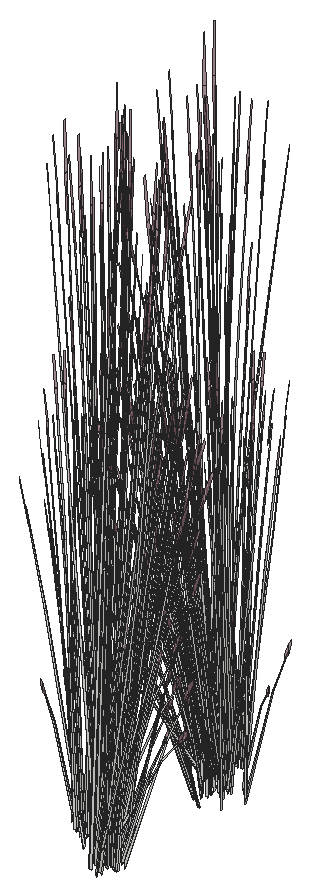
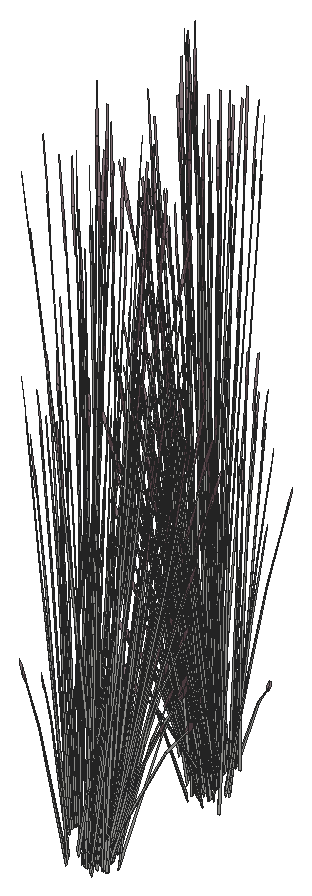
# SketchUp Ruby script. Lengths in inches.
U = 1.inch
M = Sketchup.active_model
def pt(a) = Geom::Point3d.new(a.map { |v| v * U })
def face(e, loops, mat)
  f = e.add_face(loops[0].map { |a| pt(a) })
  loops[1..].each { |l| e.add_face(l.map { |a| pt(a) }).erase! }
  f.material = f.back_material = mat if mat
  f
end
# faces: each face lists its corners as indices into pts; further lists are holes
def faces(e, pts, list, mat = nil) = list.each { |f| face(e, (f[0].is_a?(Array) ? f : [f]).map { |l| l.map { |i| pts[i] } }, mat) }
# xy, xz, yz: faces in a plane at the given z, y or x. An outline is a flat list of corners, or four numbers for a rectangle; further outlines are holes
def ring(l) = l.size == 4 ? [[l[0], l[1]], [l[2], l[1]], [l[2], l[3]], [l[0], l[3]]] : l.each_slice(2).to_a
def flat(e, list, mat, &to3) = list.each { |f| face(e, (f[0].is_a?(Array) ? f : [f]).map { |l| ring(l).map { |u, v| to3.(u, v) } }, mat) }
def xy(e, z, list, mat = nil) = flat(e, list, mat) { |x, y| [x, y, z] }
def xz(e, y, list, mat = nil) = flat(e, list, mat) { |x, z| [x, y, z] }
def yz(e, x, list, mat = nil) = flat(e, list, mat) { |y, z| [x, y, z] }
def lines(e, pts, list) = list.each { |a, b| e.add_line(pt(pts[a]), pt(pts[b])) }
# prism: a flat outline (further loops are holes) pulled along v
def prism(e, loops, v, mat = nil)
  f = face(e, loops, mat); d = Geom::Vector3d.new(v.map { |x| x * U })
  f.pushpull(f.normal.samedirection?(d) ? d.length : -d.length)
end
def box(e, o, s, mat = nil) = prism(e, [[o, [o[0] + s[0], o[1], o[2]], [o[0] + s[0], o[1] + s[1], o[2]], [o[0], o[1] + s[1], o[2]]]], [0, 0, s[2]], mat)
def at(x, y, z, deg = 0) = Geom::Transformation.translation(pt([x, y, z])) * Geom::Transformation.rotation(ORIGIN, Z_AXIS, deg.degrees)
def axes(o, x, y, z) = Geom::Transformation.new([*x, 0, *y, 0, *z, 0, *pt(o).to_a, 1])
def part(name) = M.definitions.add(name)
# library, detail: a bought-in or finely detailed component or shape, given as its bounding box
def library(name, o, s) = part(name).tap { |d| box(d.entities, o, s) }
def detail(e, o, s) = box(e.add_group.entities, o, s)
def put(e, d, t, mat = nil) = e.add_instance(d, t).tap { |i| i.material = mat if mat }
def group(e, t, mat = nil) = e.add_group.tap { |g| g.transformation = t; g.material = mat if mat }.entities
root = M.entities
M.materials.add("LightPink_Translucent").color = [144, 107, 117]
M.materials["LightPink_Translucent"].alpha = 0.75
c1 = part("blade")
p = [[2.15,0.21,22],[0,0.17,0],[0.09,0.45,0],[2.18,0.31,22],[2.29,0.31,22],[0.38,0.45,0],
  [2.48,0.24,33],[2.49,0.24,33],[2.48,0.22,33]]
faces(c1.entities,p,[[0,1,2,3],[4,5,2,3],[6,3,4,7],[8,0,3,6]])
c2 = part("seeds")
p = [[0.3,-0.1,1.38],[-0.01,-0.03,1.59],[-0.01,-0.03,0.03],[0.14,-0.07,-0.07],[0.29,-0.03,3],[0.15,0.01,3.11]]
faces(c2.entities,p,[[0,1,2,3],[1,0,4,5]],"LightPink_Translucent")
c3 = part("blade with seeds")
put(c3.entities,c1,at(0,0,0))
put(c3.entities,c2,axes([2.4,0.25,30.99],[1.5799,-0.05474,1.17369],[-0.12525,1.92788,0.29478],[-0.07173,-0.02425,1.56792]))
put(root,c3,axes([330.96,440.47,1400.67],[-0.35635,0.30962,-0.29095],[-0.23697,-0.43749,-0.50002],[-0.08792,-0.04443,1.59708]))
put(root,c3,axes([331.74,438.73,1400.47],[-0.37926,0.12378,0.17642],[-0.09365,-0.46065,0.35086],[0.03382,0.06712,1.60407]))
put(root,c3,axes([331.98,439.7,1401.875],[-0.14639,0.01056,1.71376],[0.09712,-0.45778,0.13857],[0.20862,0.02831,0.73262]))
put(root,c3,axes([332.17,438.71,1400.03],[0.08291,0.40636,-0.30978],[-0.32928,0.11539,0.30978],[0.06638,0.04686,1.38974]))
put(root,c3,axes([332.73,440.33,1402.73],[0.12963,0.31798,0.0643],[-0.23638,0.15564,0.50621],[0.1042,-0.03071,0.77189]))
put(root,c3,axes([331.5,439.62,1400.38],[-0.44609,-0.09826,0.49198],[0.09078,-0.55493,0.19306],[0.06519,0.05359,1.70813]))
put(root,c3,axes([332.71,440.22,1402.73],[-0.09971,0.42522,0.48003],[-0.32782,-0.1454,0.3958],[0.12892,-0.02555,0.9933]))
put(root,c3,axes([331.15,440.99,1400.2],[-0.11516,-0.40207,0],[0.32884,-0.1408,0],[0,0,1.54371]))
put(root,c3,axes([330.93,440.61,1400.62],[-0.06809,0.4162,0.1448],[-0.33266,-0.07225,-0.41347],[-0.06054,-0.04274,1.26744]))
put(root,c3,axes([329.64,439.53,1403.05],[0.29332,0.1301,0.35414],[-0.08555,0.37955,-0.4572],[-0.11809,0.0348,0.87481]))
put(root,c3,axes([331.58,440.93,1400.18],[0.37054,-0.15823,-0.19198],[0.1302,0.45581,0.00008],[0.0409,-0.01749,1.73897]))
put(root,c3,axes([331.71,441.12,1400.47],[0.10196,-0.46348,0.17642],[0.3731,0.13116,0.35086],[-0.06445,0.00226,1.60407]))
put(root,c3,axes([331.62,440.07,1400.21],[0.24637,0.30123,0],[-0.24637,0.30123,0],[0,0,1.69266]))
put(root,c3,axes([330.22,439.51,1401.34],[0.10032,-0.06746,1.77064],[0.0346,0.47103,0.13857],[-0.2173,0.0625,0.63284]))
put(root,c3,axes([332.29,439.94,1400.47],[-0.2773,-0.3397,0.17642],[0.27945,-0.32949,0.35086],[-0.03063,0.06937,1.60407]))
put(root,c3,axes([331.78,439.43,1400.06],[0.36714,0.07646,-0.62353],[-0.07747,0.47163,-0.16365],[0.10956,0.05715,1.37633]))
put(root,c3,axes([333.4,440.25,1400.77],[-0.21807,0.07699,1.1486],[0.10265,-0.31819,0.84392],[0.11568,0.02177,0.25299]))
put(root,c3,axes([331.07,441.17,1400.2],[-0.35581,-0.20937,0],[0.17124,-0.43505,0],[0,0,1.62707]))
put(root,c3,axes([331.36,440.61,1400.46],[-0.34464,-0.37536,-0.25192],[0.29,-0.42149,0.5513],[-0.0928,0.04391,1.68216]))
put(root,c3,axes([330.45,441.33,1400.48],[0.33032,0.23318,0.49651],[-0.19744,0.41812,0],[-0.07523,-0.05311,1.57504]))
put(root,c3,axes([331.62,439.72,1400.72],[0.17124,-0.42022,0.44739],[0.35581,0.20224,-0.21531],[0,0.09687,1.43643]))
put(root,c3,axes([333.3,441.6,1402.71],[-0.03191,-0.04083,1.77383],[0.06981,-0.43764,-0.16761],[0.12571,-0.02796,0.31391]))
put(root,c3,axes([329.14,439.82,1402.72],[-0.05763,0.06055,1.74944],[0.0049,0.44239,-0.27667],[-0.13211,0.05753,0.14031]))
put(root,c3,axes([331.55,439.96,1400.29],[0,0.53934,-0.05637],[-0.44133,0,0],[0,0.01695,1.79368]))
put(root,c3,axes([329.53,439.76,1402.68],[-0.09562,0.42421,-0.51099],[-0.32782,-0.1454,-0.3958],[-0.13199,0.0389,0.97773]))
put(root,c3,axes([329.51,439.4,1403.03],[0.17758,0.42229,-0.1216],[-0.31518,0.20752,-0.67495],[-0.13282,0.05572,1.02557]))
put(root,c3,axes([331.58,439.58,1400.21],[0.21202,0.39143,-0.44739],[-0.32115,0.27564,0.21531],[0.06861,0.04843,1.43643]))
put(root,c3,axes([333.02,441.23,1401.93],[-0.06755,-0.39203,-0.03492],[0.31928,-0.09013,-0.15832],[0.06667,0.02485,0.52218]))
put(root,c3,axes([330.26,441.58,1400.375],[-0.22066,0.46731,0],[-0.36918,-0.26061,-0.51607],[-0.08408,-0.05936,1.63711]))
put(root,c3,axes([332.19,441.22,1403.03],[0.0189,-0.47427,-0.1216],[0.35781,0.01296,-0.67495],[0.13781,0.03295,1.02557]))
put(root,c3,axes([332.52,439.95,1400.48],[0,-0.46636,0.49651],[0.39487,0,0],[0,0.10622,1.57504]))
put(root,c3,axes([331.53,440.3,1400.72],[0.38326,-0.02879,0.44739],[0.03466,0.47788,-0.21531],[-0.06861,0.04843,1.43643]))
put(root,c3,axes([331.77,439.82,1400.62],[0.32884,-0.136,0.1448],[0.11516,0.38837,-0.41347],[0,0.08547,1.26744]))
put(root,c3,axes([332.14,441.03,1403.05],[-0.20082,-0.29199,0.35414],[0.2293,-0.2764,-0.4572],[0.1165,0.04206,0.87481]))
put(root,c3,axes([331.1875,440.53,1400.21],[-0.38326,0.02879,-0.44739],[-0.03466,-0.47788,0.21531],[-0.06861,0.04843,1.43643]))
put(root,c3,axes([332.99,440.76,1400.59],[-0.085,-0.1147,1.43002],[0.1106,-0.37943,-0.30754],[0.17198,0.0514,0.61141]))
put(root,c3,axes([331.47,441.18,1400.2],[0.35581,0.20937,0],[-0.17124,0.43505,0],[0,0,1.74954]))
put(root,c3,axes([332.5,440.9375,1402.72],[0.07571,-0.00789,1.74944],[0.20767,-0.36231,-0.27667],[0.13467,0.04783,0.14031]))
put(root,c3,axes([331.61,441.64,1400.19],[-0.21791,-0.46895,-0.05142],[0.36918,-0.26061,0.51607],[-0.09097,0.04465,1.6363]))
put(root,c3,axes([331.53,440.51,1400.62],[0.26075,0.2802,0.1448],[-0.2175,0.31612,-0.41347],[-0.06054,0.04274,1.26744]))
put(root,c3,axes([329.47,440.58,1402.73],[-0.08753,-0.42921,0.48003],[0.34336,-0.07449,0.3958],[-0.1012,0.10094,0.9933]))
put(root,c3,axes([329.41,440.5,1402.73],[-0.2423,-0.19613,0.0643],[0.14107,-0.2793,0.50621],[-0.07768,0.0903,0.77189]))
put(root,c3,axes([329.52,439.98,1401.875],[0.12246,-0.09864,1.71376],[0.1031,0.45582,0.13857],[-0.19225,0.10302,0.73262]))
put(root,c3,axes([332.21,440.99,1402.98],[0.35281,0.01123,-0.71045],[-0.0237,0.47284,0.08574],[0.14947,0.0499,1.00501]))
put(root,c3,axes([331.8125,441.37,1400.48],[0.33032,-0.23318,0.49651],[0.19744,0.41812,0],[-0.07523,0.05311,1.57504]))
put(root,c3,axes([331.34,441,1400.29],[0.15345,0.53576,-0.06012],[-0.43845,0.18773,0],[0.00536,0.01871,1.72173]))
put(root,c3,axes([331.51,441.58,1400.03],[-0.32928,-0.11539,-0.30978],[0.08291,-0.40636,0.30978],[-0.06638,0.04686,1.38974]))
put(root,c3,axes([329.14,440.76,1400.59],[0.12266,0.03828,1.43002],[0.07906,0.39104,-0.30754],[-0.16661,0.0732,0.61141]))
put(root,c3,axes([329.6875,440.4375,1403.05],[0.30722,-0.06665,0.35414],[0.08112,0.381,-0.4572],[-0.08804,0.10234,0.87481]))
put(root,c3,axes([332.78,440.03,1400.375],[0.44133,0,0],[0,0.52122,-0.51607],[0,0.11871,1.63711]))
put(root,c3,axes([328.5,440.27,1402.71],[0.04504,0.01251,1.77383],[0.13934,0.41205,-0.16761],[-0.0922,0.10815,0.31391]))
put(root,c3,axes([332.61,440.3,1400.2],[-0.44111,-0.00373,-0.04976],[0,-0.52122,0.49943],[-0.01386,0.11865,1.58352]))
put(root,c3,axes([331.65,439.85,1400.67],[0.39748,0.22252,-0.29095],[-0.19139,0.46966,-0.50002],[0.01249,0.11531,1.59708]))
put(root,c3,axes([328.88,441.58,1400.77],[0.14709,-0.21136,1.1486],[0.05804,0.3346,0.84392],[-0.1063,0.05991,0.25299]))
put(root,c3,axes([332.42,441.1875,1402.53],[0.20082,0.29199,-0.35414],[-0.2293,0.2764,0.4572],[0.1165,0.04206,0.87481]))
put(root,c3,axes([332.52,440.375,1400.03],[-0.24637,0.29097,-0.30978],[-0.24637,-0.29097,0.30978],[0,0.09372,1.38974]))
put(root,c3,axes([331.46,440.4,1400.67],[0.04113,0.53214,-0.29095],[-0.42835,0.03218,-0.50002],[-0.07543,0.07088,1.59708]))
put(root,c3,axes([332.32,441.3,1402.73],[-0.01777,0.35463,0.0643],[-0.26836,-0.00972,0.50621],[0.1028,0.03711,0.77189]))
put(root,c3,axes([331.61,440.2,1400.21],[-0.17124,0.42022,-0.44739],[-0.35581,-0.20224,0.21531],[0,0.09687,1.43643]))
put(root,c3,axes([329.43,440.66,1402.53],[-0.30722,0.06665,-0.35414],[-0.08112,-0.381,0.4572],[-0.08804,0.10234,0.87481]))
put(root,c3,axes([332.34,441.1875,1402.73],[-0.26024,0.30729,0.48003],[-0.22444,-0.32634,0.3958],[0.1221,0.05668,0.9933]))
put(root,c3,axes([328.99,441.52,1403.65],[0.31145,0.12449,-0.06488],[-0.0958,0.38314,-0.29416],[-0.05094,0.05817,0.97024]))
put(root,c3,axes([331.2,440.8125,1400.06],[-0.23773,0.35053,-0.62353],[-0.29532,-0.31785,-0.16365],[-0.09526,0.08744,1.37633]))
put(root,c3,axes([331.52,441.54,1403.05],[-0.05451,-0.37564,0.35414],[0.31161,-0.09919,-0.4572],[0.0837,0.10765,0.87481]))
put(root,c3,axes([331.62,441.4,1400.33],[0.44186,0.15158,0.30756],[-0.11054,0.54181,-0.36492],[-0.07313,0.06781,1.64885]))
put(root,c3,axes([331.59,441.77,1400.02],[-0.33032,0.23318,-0.49651],[-0.19744,-0.41812,0],[-0.07523,0.05311,1.57504]))
put(root,c3,axes([332.6875,440.39,1400.02],[0,0.46636,-0.49651],[-0.39487,0,0],[0,0.10622,1.57504]))
put(root,c3,axes([331.7,440.4375,1401.875],[-0.1311,-0.08035,1.71376],[0.27131,-0.33708,0.13857],[0.16909,0.15206,0.73262]))
put(root,c3,axes([331.72,439.38,1402.47],[-0.30498,-0.24231,1.38283],[0.32203,-0.37727,0.59665],[0.0984,0.22736,1.33663]))
put(root,c3,axes([329.53,440.4,1403.03],[0.32648,0.25715,-0.1216],[-0.18809,0.3724,-0.67495],[-0.09224,0.12945,1.02557]))
put(root,c3,axes([332.18,441.35,1400.77],[-0.19872,-0.13409,1.1486],[0.2566,-0.13625,0.84392],[0.06921,0.11541,0.25299]))
put(root,c3,axes([331.49,441.74,1403.03],[0.21031,-0.39918,-0.1216],[0.30457,0.22997,-0.67495],[0.10587,0.11278,1.02557]))
put(root,c3,axes([329.97,440.29,1401.875],[0.08815,-0.14329,1.71376],[0.22258,0.38678,0.13857],[-0.15267,0.17614,0.73262]))
put(root,c3,axes([329.6875,440.71,1402.68],[0.09067,0.42583,-0.51099],[-0.34336,0.07449,-0.3958],[-0.0984,0.11438,0.97773]))
put(root,c3,axes([330.1,441.2,1403.05],[0.23881,-0.24554,0.35414],[0.22606,0.28036,-0.4572],[-0.0344,0.14245,0.87481]))
put(root,c3,axes([331.89,441.69,1400.375],[0.22066,0.46731,0],[-0.36918,0.26061,-0.51607],[-0.08408,0.05936,1.63711]))
put(root,c3,axes([331.21,442.07,1402.71],[0.00104,-0.05646,1.77383],[0.30246,-0.2491,-0.16761],[0.10506,0.08891,0.31391]))
put(root,c3,axes([332.24,441.85,1399.49],[0.02571,-0.06733,1.76342],[0.32373,-0.19829,-0.26939],[0.09815,0.10263,0.30037]))
put(root,c3,axes([331.7,439.84,1400.84],[-0.00964,-0.43909,1.41272],[0.43635,0.11382,0.59816],[-0.1032,0.24027,1.3335]))
put(root,c3,axes([331.8125,440.32,1400.09],[0.12941,0.42699,-0.69212],[-0.37279,0.15378,-0.18165],[0.0143,0.14459,1.52773]))
put(root,c3,axes([329.88,441.42,1402.73],[-0.29004,-0.02173,0.0643],[0.00795,-0.32812,0.50621],[-0.03035,0.12569,0.77189]))
put(root,c3,axes([329.27,441.79,1399.49],[0.04734,0.04659,1.76342],[0.08027,0.4317,-0.26939],[-0.10492,0.09206,0.30037]))
put(root,c3,axes([329.98,441.45,1402.73],[-0.25132,-0.3182,0.48003],[0.2669,-0.27442,0.3958],[-0.04636,0.14929,0.9933]))
put(root,c3,axes([331.74,441.54,1402.68],[0.34827,-0.11086,-0.51099],[0.06092,0.41983,-0.3958],[0.09354,0.12031,0.97773]))
put(root,c3,axes([330.77,441.6,1403.05],[0.1064,-0.35863,0.35414],[0.31043,0.1046,-0.4572],[0.02846,0.14439,0.87481]))
put(root,c3,axes([332.22,441.96,1400.67],[-0.22633,-0.01463,1.0506],[0.14947,-0.31064,0.58006],[0.08941,0.11036,0.8241]))
put(root,c3,axes([331.56,441.88,1402.73],[-0.16041,0.29625,0.0643],[-0.22843,-0.17248,0.50621],[0.07385,0.09498,0.77189]))
put(root,c3,axes([331.1875,442.88,1403.65],[0.2439,-0.26754,-0.06488],[0.22348,0.29302,-0.29416],[0.01573,0.08303,0.97024]))
put(root,c3,axes([331.63,441.8,1402.73],[-0.35104,0.10702,0.48003],[-0.06092,-0.41983,0.3958],[0.08256,0.12373,0.9933]))
put(root,c3,axes([329.9,440.64,1401.875],[0.06572,-0.16029,1.71376],[0.27569,0.33172,0.13857],[-0.12437,0.20675,0.73262]))
put(root,c3,axes([331.48,441.21,1400.59],[0.00623,-0.15459,1.43002],[0.29764,-0.17268,-0.30754],[0.09188,0.18503,0.61141]))
put(root,c3,axes([330.67,441.93,1402.73],[-0.26007,0.1585,0.0643],[-0.12729,-0.28902,0.50621],[0.02512,0.1274,0.77189]))
put(root,c3,axes([329.98,441.55,1402.53],[-0.23881,0.24554,-0.35414],[-0.22606,-0.28036,0.4572],[-0.0344,0.14245,0.87481]))
put(root,c3,axes([329.15,441.47,1402.72],[-0.00877,0.09229,1.74944],[0.24897,0.32105,-0.27667],[-0.06518,0.15182,0.14031]))
put(root,c3,axes([329.95,441.26,1403.4],[0.3879,0.02311,-0.13498],[-0.0106,0.43749,-0.74919],[-0.02694,0.1685,1.13838]))
put(root,c3,axes([330.67,441.75,1403.03],[0.34538,-0.21713,-0.1216],[0.16972,0.38536,-0.67495],[0.04557,0.16239,1.02557]))
put(root,c3,axes([330.77,441.9,1403.0625],[-0.34777,-0.12192,0.53283],[0.11892,-0.40083,0.43934],[0.0209,0.15763,1.10256]))
put(root,c3,axes([330.13,442.5,1400.77],[-0.00913,-0.2773,1.1486],[0.22824,0.19778,0.84392],[-0.04489,0.13217,0.25299]))
put(root,c3,axes([330.73,441.84,1399.49],[0.05712,-0.02538,1.76342],[0.34359,0.13968,-0.26939],[0.01005,0.15742,0.30037]))
put(root,c3,axes([330.21,441.43,1403],[0.25266,0.31335,-0.5672],[-0.2669,0.27442,-0.43934],[-0.03844,0.15921,1.08528]))
put(root,c3,axes([329.9375,441.9,1400.82],[0.32063,-0.08258,0.06507],[0.07371,0.33271,-0.86304],[-0.02033,0.16842,0.7736]))
put(root,c3,axes([330.96,441.73,1402.68],[0.34695,0.11691,-0.51099],[-0.11892,0.40083,-0.3958],[0.03181,0.16138,0.97773]))
put(root,c3,axes([331.16,440.91,1401.875],[-0.08068,-0.14973,1.71376],[0.3728,-0.12606,0.13857],[0.08426,0.23506,0.73262]))
put(root,c3,axes([330.8,441.98,1402.53],[-0.1064,0.35863,-0.35414],[-0.31043,-0.1046,0.4572],[0.02846,0.14439,0.87481]))
put(root,c3,axes([330.13,441.29,1403.34],[-0.00918,0.43138,-0.7886],[-0.38672,-0.02897,0.09517],[-0.04081,0.18275,1.11556]))
put(root,c3,axes([329.125,442.42,1402.71],[0.04004,-0.02816,1.77383],[0.33095,0.18728,-0.16761],[-0.00778,0.15594,0.31391]))
put(root,c3,axes([330.5,440.98,1401.875],[-0.00864,-0.17899,1.71376],[0.37441,0.11874,0.13857],[-0.02316,0.25508,0.73262]))
put(root,c3,axes([330.84,441.66,1402.98],[0.16845,0.3792,-0.71045],[-0.34676,0.21133,0.08574],[0.03939,0.18322,1.00501]))
put(root,c3,axes([329.86,442.25,1400.59],[0.11138,-0.07357,1.43002],[0.27499,0.22183,-0.30754],[-0.08185,0.19194,0.61141]))
put(root,c3,axes([330.58,442.61,1402.72],[0.04474,0.0751,1.74944],[0.36104,0.0295,-0.27667],[0.03631,0.16562,0.14031]))
put(root,c3,axes([330.01,441.89,1401.36],[0.00775,-0.24075,1.54345],[0.34877,0.12716,0.21329],[-0.03022,0.25658,0.72882]))
put(root,c3,axes([330.27,453.03,1401.875],[0.08068,0.14973,1.71376],[-0.3728,0.12606,0.13857],[-0.08426,-0.23506,0.73262]))
put(root,c3,axes([330.89,452.04,1402.72],[-0.05398,-0.06539,1.74944],[-0.36026,0.04145,-0.27667],[-0.0575,-0.15639,0.14031]))
put(root,c3,axes([331.72,452.82,1400.59],[-0.10032,0.0944,1.43002],[-0.30046,-0.16522,-0.30754],[0.05569,-0.20547,0.61141]))
put(root,c3,axes([331.27,453.15,1402.98],[-0.16845,-0.3792,-0.71045],[0.34676,-0.21133,0.08574],[-0.03939,-0.18322,1.00501]))
put(root,c3,axes([330.17,452.64,1400.59],[-0.02137,0.15256,1.43002],[-0.31245,0.12771,-0.30754],[-0.07303,-0.19719,0.61141]))
put(root,c3,axes([330.98,452.3,1399.49],[-0.0592,0.0168,1.76342],[-0.32738,-0.18913,-0.26939],[0.00549,-0.15776,0.30037]))
put(root,c3,axes([331.97,453.52,1402.98],[0.00918,-0.43138,-0.71045],[0.38672,0.02897,0.08574],[0.04081,-0.18275,1.00501]))
put(root,c3,axes([332.51,452.84,1402.72],[-0.00341,-0.09282,1.74944],[-0.28775,-0.26825,-0.27667],[0.04449,-0.16261,0.14031]))
put(root,c3,axes([331.3,452.82,1402.53],[0.1064,-0.35863,-0.35414],[0.31043,0.1046,0.4572],[-0.02846,-0.14439,0.87481]))
put(root,c3,axes([331.53,453.3,1401.875],[-0.06572,0.16029,1.71376],[-0.27569,-0.33172,0.13857],[0.12437,-0.20675,0.73262]))
put(root,c3,axes([332.43,452.51,1402.71],[-0.03584,0.03562,1.77383],[-0.35118,-0.12018,-0.16761],[-0.01271,-0.15545,0.31391]))
put(root,c3,axes([331.14,453.07,1402.68],[-0.34695,-0.11691,-0.51099],[0.11892,-0.40083,-0.3958],[-0.03181,-0.16138,0.97773]))
put(root,c3,axes([331.35,452.07,1400.77],[0.04528,0.27194,1.1486],[-0.25117,-0.15062,0.84392],[0.02703,-0.13924,0.25299]))
put(root,c3,axes([331.89,453.375,1402.68],[-0.25266,-0.31335,-0.51099],[0.2669,-0.27442,-0.3958],[0.03844,-0.15921,0.97773]))
put(root,c3,axes([330.52,451.83,1402.71],[-0.00658,0.0559,1.77383],[-0.32474,0.20287,-0.16761],[-0.09556,-0.1037,0.31391]))
put(root,c3,axes([330.45,452.82,1403.09],[0.39316,-0.11987,0.53763],[0.06823,0.47021,0.4433],[-0.09247,-0.13858,1.11249]))
put(root,c3,axes([331.34,452.91,1402.73],[0.34777,0.12192,0.48003],[-0.11892,0.40083,0.3958],[-0.0209,-0.15763,0.9933]))
put(root,c3,axes([331.4375,453.05,1403.03],[-0.34538,0.21713,-0.1216],[-0.16972,-0.38536,-0.67495],[-0.04557,-0.16239,1.02557]))
put(root,c3,axes([332.15,453.54,1403.03],[-0.3879,-0.02311,-0.1216],[0.0106,-0.43749,-0.67495],[0.02694,-0.1685,1.02557]))
put(root,c3,axes([332.13,453.26,1402.53],[0.23881,-0.24554,-0.35414],[0.22606,0.28036,0.4572],[0.0344,-0.14245,0.87481]))
put(root,c3,axes([330.0625,452.39,1400.77],[0.18411,0.16231,1.1486],[-0.26813,0.09757,0.84392],[-0.05737,-0.12474,0.25299]))
put(root,c3,axes([331.43,452.875,1402.73],[0.26007,-0.1585,0.0643],[0.12729,0.28902,0.50621],[-0.02512,-0.1274,0.77189]))
put(root,c3,axes([330.51,453.25,1402.98],[-0.30095,-0.22541,-0.71045],[0.21388,-0.395,0.08574],[-0.10904,-0.13459,1.00501]))
put(root,c3,axes([330.4,452.95,1402.53],[-0.05451,-0.37564,-0.35414],[0.31161,-0.09919,0.4572],[-0.0837,-0.10765,0.87481]))
put(root,c3,axes([330.54,452.92,1402.73],[0.16041,-0.29625,0.0643],[0.22843,0.17248,0.50621],[-0.07385,-0.09498,0.77189]))
put(root,c3,axes([329.92,452.88,1399.49],[-0.03419,0.06144,1.76342],[-0.3455,0.13246,-0.26939],[-0.08346,-0.12049,0.30037]))
put(root,c3,axes([330.49,454.57,1400.1],[-0.14494,-0.47823,-0.69835],[0.41752,-0.17223,-0.18329],[-0.01602,-0.16194,1.54149]))
put(root,c3,axes([329.73,453.5,1401.875],[0.1311,0.08035,1.71376],[-0.27131,0.33708,0.13857],[-0.16909,-0.15206,0.73262]))
put(root,c3,axes([332.43,453.11,1399.49],[-0.05283,-0.03674,1.76342],[-0.13569,-0.41045,-0.26939],[0.09154,-0.11138,0.30037]))
put(root,c3,axes([331.33,453.2,1403.05],[-0.1064,0.35863,0.35414],[-0.31043,-0.1046,-0.4572],[-0.02846,-0.14439,0.87481]))
put(root,c3,axes([330.37,453.26,1402.68],[-0.34827,0.11086,-0.51099],[-0.06092,-0.41983,-0.3958],[-0.09354,-0.12031,0.97773]))
put(root,c3,axes([332.125,453.35,1402.73],[0.25132,0.3182,0.48003],[-0.2669,0.27442,0.3958],[0.04636,-0.14929,0.9933]))
put(root,c3,axes([330.61,452.89,1403.43],[-0.23555,0.44708,-0.13619],[-0.34112,-0.25757,-0.75594],[-0.11858,-0.12631,1.14864]))
put(root,c3,axes([332.22,453.38,1402.73],[0.29004,0.02173,0.0643],[-0.00795,0.32812,0.50621],[0.03035,-0.12569,0.77189]))
put(root,c3,axes([332,453.61,1403.05],[-0.23881,0.24554,0.35414],[-0.22606,-0.28036,-0.4572],[0.0344,-0.14245,0.87481]))
put(root,c3,axes([332.42,454.27,1402.98],[0.18436,-0.36797,-0.71045],[0.32306,0.26151,0.08574],[0.11008,-0.13332,1.00501]))
put(root,c3,axes([330.43,453.19,1400.375],[-0.22066,-0.46731,0],[0.36918,-0.26061,-0.51607],[0.08408,-0.05936,1.63711]))
put(root,c3,axes([332.41,454.09,1402.68],[-0.09067,-0.42583,-0.51099],[0.34336,-0.07449,-0.3958],[0.0984,-0.11438,0.97773]))
put(root,c3,axes([330.92,452.63,1400.13],[-0.2439,0.26754,-0.03893],[-0.22348,-0.29302,-0.17649],[-0.01573,-0.08303,0.58215]))
put(root,c3,axes([329.71,452.76,1402.72],[-0.07594,-0.00329,1.74944],[-0.24177,0.32918,-0.27667],[-0.129,-0.06726,0.14031]))
put(root,c3,axes([332.58,454.4,1403.03],[-0.32648,-0.25715,-0.1216],[0.18809,-0.3724,-0.67495],[0.09224,-0.12945,1.02557]))
put(root,c3,axes([331.23,455.8,1401.33],[0.305,0.18805,1.51261],[-0.29879,0.40513,0.59816],[-0.13384,-0.24012,1.26806]))
put(root,c3,axes([330.59,453.26,1403.05],[0.05451,0.37564,0.35414],[-0.31161,0.09919,-0.4572],[-0.0837,-0.10765,0.87481]))
put(root,c3,axes([329.63,454.5,1400.02],[0,-0.46636,-0.49651],[0.39487,0,0],[0,-0.10622,1.57504]))
put(root,c3,axes([330.73,453.12,1400.02],[0.33032,-0.23318,-0.49651],[0.19744,0.41812,0],[0.07523,-0.05311,1.57504]))
put(root,c3,axes([332.69,453.93,1400.59],[-0.12609,-0.01381,1.43002],[-0.12917,-0.37055,-0.30754],[0.1549,-0.10482,0.61141]))
put(root,c3,axes([329.65,453.51,1403.09],[0.29147,-0.34417,0.53763],[0.25138,0.3655,0.4433],[-0.13675,-0.06349,1.11249]))
put(root,c3,axes([333.38,454.29,1402.71],[-0.0461,-0.00354,1.77383],[-0.19143,-0.37951,-0.16761],[0.07688,-0.12478,0.31391]))
put(root,c3,axes([331.12,454.08,1400.06],[0.23773,-0.35053,-0.62353],[0.29532,0.31785,-0.16365],[0.09526,-0.08744,1.37633]))
put(root,c3,axes([332.84,453.25,1400.77],[-0.11756,0.2374,1.1486],[-0.10105,-0.31895,0.84392],[0.09709,-0.07992,0.25299]))
put(root,c3,axes([332.67,454.14,1402.53],[0.30722,-0.06665,-0.35414],[0.08112,0.381,0.4572],[0.08804,-0.10234,0.87481]))
put(root,c3,axes([329.78,453.5,1402.73],[0.01777,-0.35463,0.0643],[0.26836,0.00972,0.50621],[-0.1028,-0.03711,0.77189]))
put(root,c3,axes([330.71,454.69,1400.21],[0.17124,-0.42022,-0.44739],[0.35581,0.20224,0.21531],[0,-0.09687,1.43643]))
put(root,c3,axes([329.68,453.62,1402.53],[-0.20082,-0.29199,-0.35414],[0.2293,-0.2764,0.4572],[-0.1165,-0.04206,0.87481]))
put(root,c3,axes([330.86,454.49,1400.67],[-0.04113,-0.53214,-0.29095],[0.42835,-0.03218,-0.50002],[0.07543,-0.07088,1.59708]))
put(root,c3,axes([329.8,454.51,1400.03],[0.24637,-0.29097,-0.30978],[0.24637,0.29097,0.30978],[0,-0.09372,1.38974]))
put(root,c3,axes([329.7,453.12,1400.13],[-0.10181,0.3808,-0.03893],[-0.31336,-0.11714,-0.17649],[-0.04758,-0.06228,0.58215]))
put(root,c3,axes([332.42,454.36,1403.05],[-0.30722,0.06665,0.35414],[-0.08112,-0.381,-0.4572],[0.08804,-0.10234,0.87481]))
put(root,c3,axes([330.67,455.04,1400.67],[-0.39748,-0.22252,-0.29095],[0.19139,-0.46966,-0.50002],[-0.01249,-0.11531,1.59708]))
put(root,c3,axes([329.53,454.86,1400.375],[-0.44133,0,0],[0,-0.52122,-0.51607],[0,-0.11871,1.63711]))
put(root,c3,axes([329.61,453.93,1400.59],[0.06891,0.12984,1.43002],[-0.15879,0.35293,-0.30754],[-0.16304,-0.08436,0.61141]))
put(root,c3,axes([330.81,453.31,1400.03],[0.32928,0.11539,-0.30978],[-0.08291,0.40636,0.30978],[0.06638,-0.04686,1.38974]))
put(root,c3,axes([329.89,453.81,1402.98],[-0.35281,-0.01123,-0.71045],[0.0237,-0.47284,0.08574],[-0.14947,-0.0499,1.00501]))
put(root,c3,axes([332.7,454.3,1402.73],[0.2423,0.19613,0.0643],[-0.14107,0.2793,0.50621],[0.07768,-0.0903,0.77189]))
put(root,c3,axes([332.63,454.22,1402.73],[0.08753,0.42921,0.48003],[-0.34336,0.07449,0.3958],[0.1012,-0.10094,0.9933]))
put(root,c3,axes([333.55,454.74,1402.72],[0.04898,-0.07104,1.74944],[-0.06269,-0.43574,-0.27667],[0.12289,-0.08262,0.14031]))
put(root,c3,axes([329.875,454.72,1400.33],[-0.32829,0.39208,0.30756],[-0.32849,-0.38796,-0.36492],[-0.01146,-0.11134,1.64885]))
put(root,c3,axes([329.42,453.04,1402.71],[0.02617,0.04654,1.77383],[-0.12614,0.41836,-0.16761],[-0.12775,0.00303,0.31391]))
put(root,c3,axes([330.92,454.9,1400.43],[0.39767,0.22603,0.24065],[-0.19139,0.46966,0.50002],[0,-0.10827,1.60543]))
put(root,c3,axes([330.77,455.54,1400.4375],[0.09355,-0.55261,-0.23429],[0.44354,0.09633,0.51271],[-0.0775,-0.07631,1.5644]))
put(root,c3,axes([329.78,453.91,1402.68],[-0.25628,0.30892,-0.51099],[-0.22444,-0.32634,-0.3958],[-0.13021,-0.047,0.97773]))
put(root,c3,axes([329.97,453.77,1403.05],[0.20082,0.29199,0.35414],[-0.2293,0.2764,-0.4572],[-0.1165,-0.04206,0.87481]))
put(root,c3,axes([329.2,454.32,1400.77],[0.22533,-0.03337,1.1486],[-0.14293,0.29403,0.84392],[-0.11135,-0.04411,0.25299]))
put(root,c3,axes([330.79,454.59,1400.72],[-0.38326,0.02879,0.44739],[-0.03466,-0.47788,-0.21531],[0.06861,-0.04843,1.43643]))
put(root,c3,axes([329.91,453.58,1403.03],[-0.0189,0.47427,-0.1216],[-0.35781,-0.01296,-0.67495],[-0.13781,-0.03295,1.02557]))
put(root,c3,axes([329.8,454.9375,1400.48],[0,0.46636,0.49651],[-0.39487,0,0],[0,-0.10622,1.57504]))
put(root,c3,axes([332.59,455.4,1403.03],[-0.17758,-0.42229,-0.1216],[0.31518,-0.20752,-0.67495],[0.13282,-0.05572,1.02557]))
put(root,c3,axes([332.57,455.04,1402.68],[0.09562,-0.42421,-0.51099],[0.32782,0.1454,-0.3958],[0.13199,-0.0389,0.97773]))
put(root,c3,axes([332.06,453.3125,1400.375],[0.22066,-0.46731,0],[0.36918,0.26061,-0.51607],[0.08408,0.05936,1.63711]))
put(root,c3,axes([329.46,454.24,1401.875],[0.14639,-0.01056,1.71376],[-0.09712,0.45778,0.13857],[-0.20862,-0.02831,0.73262]))
put(root,c3,axes([330.73,455.3125,1400.21],[-0.21202,-0.39143,-0.44739],[0.32115,-0.27564,0.21531],[-0.06861,-0.04843,1.43643]))
put(root,c3,axes([330.78,454.76,1400.36],[0.15345,0.52148,0.45755],[-0.43845,0.18134,0.17955],[0.00536,-0.09582,1.58856]))
put(root,c3,axes([332.92,455.16,1399.98],[-0.22732,0.05597,1.41583],[-0.03618,-0.44548,0.08104],[0.15921,-0.06743,0.80566]))
put(root,c3,axes([333.34,454.76,1400.26],[-0.21881,-0.29821,-0.06488],[0.23965,-0.27324,-0.29416],[0.0679,-0.01924,0.97024]))
put(root,c3,axes([330.7,455.17,1400.72],[-0.17124,0.42022,0.44739],[-0.35581,-0.20224,-0.21531],[0,-0.09687,1.43643]))
put(root,c3,axes([331.33,454.8,1400.21],[0,-0.53961,0],[0.44133,0,0],[0,0,1.79456]))
put(root,c3,axes([331.87,453.56,1400.48],[-0.33032,-0.23318,0.49651],[0.19744,-0.41812,0],[0.07523,0.05311,1.57504]))
put(root,c3,axes([332.51,455.19,1402.98],[0.31014,-0.20596,-0.71045],[0.17284,0.42397,0.08574],[0.14985,-0.04816,1.00501]))
put(root,c3,axes([330.54,455.46,1400.06],[-0.36714,-0.07646,-0.62353],[0.07747,-0.47163,-0.16365],[-0.10956,-0.05715,1.37633]))
put(root,c3,axes([331.12,454.46,1400.36],[-0.29264,0.42323,0.45755],[-0.34767,-0.3736,0.17955],[0.07055,-0.04224,1.58856]))
put(root,c3,axes([331.44,455.22,1400.3],[-0.32829,-0.4014,-0.06131],[0.32849,-0.40164,0],[-0.01146,-0.01402,1.75571]))
put(root,c3,axes([330.61,453.77,1400.47],[-0.10196,0.46348,0.17642],[-0.3731,-0.13116,0.35086],[0.06445,-0.00226,1.60407]))
put(root,c3,axes([332.47,455.28,1403.05],[-0.29332,-0.1301,0.35414],[0.08555,-0.37955,-0.4572],[0.11809,-0.0348,0.87481]))
put(root,c3,axes([329.4,454.58,1402.73],[0.09971,-0.42522,0.48003],[0.32782,0.1454,0.3958],[-0.12892,0.02555,0.9933]))
put(root,c3,axes([330.46,454.14,1399.59],[-0.3474,0.18671,1.28929],[-0.11057,-0.53572,0.50096],[0.21332,0.00891,1.46642]))
put(root,c3,axes([331.39,454.28,1400.62],[0.06809,-0.4162,0.1448],[0.33266,0.07225,-0.41347],[0.06054,0.04274,1.26744]))
put(root,c3,axes([329.37,454.47,1402.73],[-0.12963,-0.31798,0.0643],[0.23638,-0.15564,0.50621],[-0.1042,0.03071,0.77189]))
put(root,c3,axes([330.82,455.27,1400.36],[0.44609,0.09826,0.45755],[-0.09078,0.55493,0.17955],[-0.06519,-0.05359,1.58856]))
put(root,c3,axes([333.17,454.87,1399.49],[-0.01845,-0.0708,1.76342],[0.12793,-0.41416,-0.26939],[0.12905,-0.00596,0.30037]))
